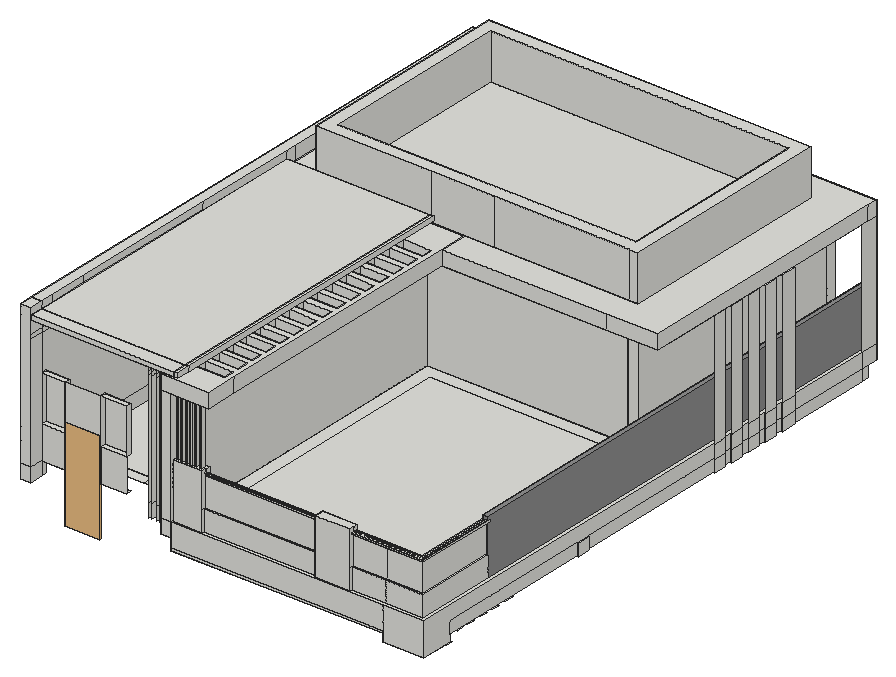
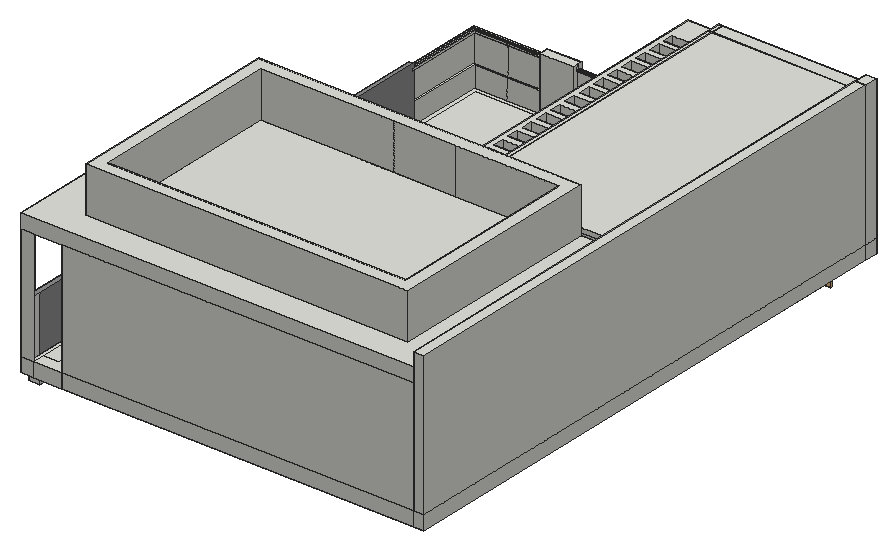
# SketchUp Ruby script. Lengths in inches.
U = 1.inch
M = Sketchup.active_model
def pt(a) = Geom::Point3d.new(a.map { |v| v * U })
def face(e, loops, mat)
  f = e.add_face(loops[0].map { |a| pt(a) })
  loops[1..].each { |l| e.add_face(l.map { |a| pt(a) }).erase! }
  f.material = f.back_material = mat if mat
  f
end
# faces: each face lists its corners as indices into pts; further lists are holes
def faces(e, pts, list, mat = nil) = list.each { |f| face(e, (f[0].is_a?(Array) ? f : [f]).map { |l| l.map { |i| pts[i] } }, mat) }
# xy, xz, yz: faces in a plane at the given z, y or x. An outline is a flat list of corners, or four numbers for a rectangle; further outlines are holes
def ring(l) = l.size == 4 ? [[l[0], l[1]], [l[2], l[1]], [l[2], l[3]], [l[0], l[3]]] : l.each_slice(2).to_a
def flat(e, list, mat, &to3) = list.each { |f| face(e, (f[0].is_a?(Array) ? f : [f]).map { |l| ring(l).map { |u, v| to3.(u, v) } }, mat) }
def xy(e, z, list, mat = nil) = flat(e, list, mat) { |x, y| [x, y, z] }
def xz(e, y, list, mat = nil) = flat(e, list, mat) { |x, z| [x, y, z] }
def yz(e, x, list, mat = nil) = flat(e, list, mat) { |y, z| [x, y, z] }
def lines(e, pts, list) = list.each { |a, b| e.add_line(pt(pts[a]), pt(pts[b])) }
# prism: a flat outline (further loops are holes) pulled along v
def prism(e, loops, v, mat = nil)
  f = face(e, loops, mat); d = Geom::Vector3d.new(v.map { |x| x * U })
  f.pushpull(f.normal.samedirection?(d) ? d.length : -d.length)
end
def box(e, o, s, mat = nil) = prism(e, [[o, [o[0] + s[0], o[1], o[2]], [o[0] + s[0], o[1] + s[1], o[2]], [o[0], o[1] + s[1], o[2]]]], [0, 0, s[2]], mat)
def at(x, y, z, deg = 0) = Geom::Transformation.translation(pt([x, y, z])) * Geom::Transformation.rotation(ORIGIN, Z_AXIS, deg.degrees)
def axes(o, x, y, z) = Geom::Transformation.new([*x, 0, *y, 0, *z, 0, *pt(o).to_a, 1])
def part(name) = M.definitions.add(name)
# library, detail: a bought-in or finely detailed component or shape, given as its bounding box
def library(name, o, s) = part(name).tap { |d| box(d.entities, o, s) }
def detail(e, o, s) = box(e.add_group.entities, o, s)
def put(e, d, t, mat = nil) = e.add_instance(d, t).tap { |i| i.material = mat if mat }
def group(e, t, mat = nil) = e.add_group.tap { |g| g.transformation = t; g.material = mat if mat }.entities
root = M.entities
M.materials.add("[Color M04]").color = [142, 142, 142]
c1 = library("c103.dxf",[0,0,0],[4.7,1.18,0.06])
xy(root,216,[[117,47.75,165,56.75],[201,47.75,261,56.75],[306,160,315,220],[306,256,315,304],[306,393.91,315,441.91]])
xy(root,235.625,[[315,0,315,9.8125,341.1875,9.8125,341.1875,28.05,341.78,28.05,341.78,23.68,351,23.68,351,0],[341.78,23.68,351,28.05],[351,23.68,352.3125,23.68,352.3125,28.93,341.78,28.93,341.78,28.05,351,28.05]])
xy(root,241.9375,[[341.1875,28.05,341.1875,482.75,351,482.75,351,401.04,352.3125,401.04,352.3125,388.24,351,388.24,351,380.51,352.3125,380.51,352.3125,369.53,351,369.53,351,362.89,352.3125,362.89,352.3125,351.72,351,351.72,351,343.76,352.3125,343.76,352.3125,332.62,351,332.62,351,325.96,352.3125,325.96,352.3125,314.875,351,314.875,351,177.375,352.3125,177.375,352.3125,166.56,351,166.56,351,94.89,341.78,94.89,341.78,87.35,351,87.35,351,79.37,341.78,79.37,341.78,73.23,351,73.23,351,66.7,341.78,66.7,341.78,60.24,351,60.24,351,52.82,341.78,52.82,341.78,46.18,351,46.18,351,41.08,341.78,41.08,341.78,35.09,351,35.09,351,28.05],[341.78,35.09,351,41.08],[351,35.09,352.3125,41.08],[341.78,46.18,351,52.82],[351,46.18,352.3125,52.82],
  [341.78,60.24,351,66.7],[351,60.24,352.3125,66.7],[341.78,73.23,351,79.37],[351,73.23,352.3125,79.37],[341.78,87.35,351,94.89],
  [351,87.35,352.3125,94.89]])
xy(root,242,[[131.25,0,315,9.8125]])
xy(root,244,[[131.25,0,315,9.8125]])
xy(root,252,[[0,0,9,11.75],[122.25,0,131.25,11.75],[131.25,9.8125,131.25,11.75,132.375,11.75,132.375,22.5,131.25,22.5,131.25,47.75,315,47.75,315,482.75,341.1875,482.75,341.1875,472.9375,324.8125,472.9375,324.8125,37.9375,141.0625,37.9375,141.0625,32.3125,142.1875,32.3125,142.1875,9.8125],[142.1875,9.8125,142.1875,32.3125,141.0625,32.3125,141.0625,37.9375,324.8125,37.9375,324.8125,472.9375,341.1875,472.9375,341.1875,9.8125],[122.25,11.75,125.16,16.5625],
  [131.25,11.75,132.375,22.5],[341.1875,28.05,351,28.05,351,314.875,352.3125,314.875,352.3125,325.96,351,325.96,351,332.62,352.3125,332.62,352.3125,343.76,351,343.76,351,351.72,352.3125,351.72,352.3125,362.89,351,362.89,351,369.53,352.3125,369.53,352.3125,380.51,351,380.51,351,388.24,352.3125,388.24,352.3125,401.04,351,401.04,351,482.75,341.1875,482.75],[0,47.75,69,56.75],[69,47.75,131.25,56.75],[131.25,47.75,315,56.75],
  [0,56.75,69,56.81],[69,56.75,78,482.75],[78,56.75,78,482.75,306,482.75,306,278.1875,131.25,278.1875,131.25,56.75],[131.25,56.75,306,278.1875],[306,56.75,315,278.1875],
  [0,56.81,69,187.47],[351,166.56,352.3125,177.375],[0,187.47,69,482.75],[306,278.1875,315,482.75],[0,482.75,69,491.75],
  [69,482.75,315,491.75],[315,482.75,351,491.75]])
xy(root,252.9375,[[341.78,166.56,345.03,166.56,341.78,177.375]])
xy(root,264,[[0,0,9,11.75],[122.25,0,131.25,11.75],[131.25,0,351,0,351,314.875,352.3125,314.875,352.3125,325.96,351,325.96,351,332.62,352.3125,332.62,352.3125,343.76,351,343.76,351,351.72,352.3125,351.72,352.3125,362.89,351,362.89,351,369.53,352.3125,369.53,352.3125,380.51,351,380.51,351,388.24,352.3125,388.24,352.3125,401.04,351,401.04,351,491.75,339.5,491.75,339.5,11.5,143.875,11.5,132.375,11.75,131.25,11.75,131.25,8.15,143.83,7.95,143.83,9.89,156.7,9.89,156.7,7.95,255.15,7.95,255.15,9.89,285.07,9.89,285.07,7.95,343.05,7.95,343.05,488.2,347.45,488.2,347.45,3.55,285.07,3.55,285.07,1.61,255.15,1.61,255.15,3.55,156.7,3.55,156.7,1.61,131.25,1.61],[131.25,1.61,131.25,8.15,143.83,7.95,143.83,9.89,156.7,9.89,156.7,7.95,255.15,7.95,255.15,9.89,285.07,9.89,285.07,7.95,343.05,7.95,343.05,73.86,347.45,73.86,347.45,3.55,285.07,3.55,285.07,1.61,255.15,1.61,255.15,3.55,156.7,3.55,156.7,1.61],[143.875,11.5,143.875,34,142.75,34,142.75,266.6875,326.5,266.6875,326.5,480.25,339.5,480.25,339.5,491.75,315,491.75,315,278.1875,131.25,278.1875,131.25,22.5,132.375,22.5,132.375,11.75],
  [143.875,11.5,339.5,11.5,339.5,480.25,326.5,480.25,326.5,266.6875,142.75,266.6875,142.75,34,143.875,34],[9,11.75,29.4,16.5625],[60.19,11.75,82.8125,16.5625],[122.25,11.75,131.25,22.5],[131.25,11.75,132.375,22.5],
  [122.25,22.5,131.25,278.1875],[343.05,73.86,347.45,488.2],[9,278.1875,306,287.1875],[306,278.1875,315,482.75],[9,482.75,315,491.75]])
xy(root,282,[[156.7,3.55,255.15,5.09],[285.07,3.55,347.45,3.55,347.45,73.86,345.91,73.86,345.91,5.09,285.07,5.09],[156.7,6.41,255.15,7.95],[285.07,6.41,344.59,6.41,344.59,73.86,343.05,73.86,343.05,7.95,285.07,7.95]])
xy(root,292.85,[[9,11.75,29.4,16.5625],[60.19,11.75,82.8125,16.5625]])
xy(root,307.3125,[[[283.34,3.36,283.34,8.14,342.86,8.14,342.86,75.59,347.64,75.59,347.64,3.36],[285.07,5.09,345.91,5.09,345.91,73.86,344.59,73.86,344.59,6.41,285.07,6.41]],[[155.89,4.28,255.96,7.22],[156.7,5.09,255.15,6.41]],[156.7,5.09,255.15,6.41],[285.07,5.09,285.07,6.41,344.59,6.41,344.59,73.86,345.91,73.86,345.91,5.09]])
xy(root,308.625,[[[283.34,3.36,347.64,3.36,347.64,75.59,342.86,75.59,342.86,8.14,283.34,8.14],[285.07,5.09,285.07,6.41,344.59,6.41,344.59,73.86,345.91,73.86,345.91,5.09]],[[155.89,4.28,255.96,7.22],[156.7,5.09,255.15,6.41]],[156.7,5.09,255.15,6.41],[285.07,5.09,345.91,5.09,345.91,73.86,344.59,73.86,344.59,6.41,285.07,6.41]])
xy(root,312,[[[131.25,1.61,156.7,1.61,156.7,9.89,143.83,9.89,143.83,7.95,131.25,8.15],[132.875,3.73,135.0625,7.27],[136.5,3.73,138.6875,7.27],[140.5625,3.73,142.75,7.27],[144.5,3.73,146.6875,7.27],[148.5,3.73,150.6875,7.27],[152.875,3.73,155.0625,7.27]],[255.15,1.61,285.07,9.89],[132.875,3.73,135.0625,7.27],[136.5,3.73,138.6875,7.27],[140.5625,3.73,142.75,7.27],
  [144.5,3.73,146.6875,7.27],[148.5,3.73,150.6875,7.27],[152.875,3.73,155.0625,7.27]])
xy(root,312,[[343.05,73.86,347.45,488.2]],"[Color M04]")
xy(root,332.24,[[9,11.75,29.4,16.5625],[60.19,11.75,82.8125,16.5625]])
xy(root,363.8125,[[122.25,0,131.25,278.1875],[[131.25,0,131.25,27.62,133.86,27.62,133.86,23.53,158.62,23.53,158.62,27.62,163.5625,27.62,163.5625,0],[152.875,3.73,155.0625,7.27],[144.5,3.73,146.6875,7.27],[148.5,3.73,150.6875,7.27],[140.5625,3.73,142.75,7.27],[136.5,3.73,138.6875,7.27],[132.875,3.73,135.0625,7.27]],[[131.25,27.62,131.25,278.1875,163.5625,278.1875,163.5625,27.62,158.62,27.62,158.62,33.15,133.86,33.15,133.86,27.62],[133.86,38.59,158.62,48.21],[133.86,53.65,158.62,63.28],[133.86,68.71,158.62,78.34],[133.86,83.78,158.62,93.4],[133.86,99.28,158.62,108.9],[133.86,114.78,158.62,124.4],[133.86,223.28,158.62,232.9],[133.86,207.78,158.62,217.4],[133.86,176.78,158.62,186.4],[133.86,130.28,158.62,139.9],[133.86,161.28,158.62,170.9],[133.86,238.78,158.62,248.4],[133.86,192.28,158.62,201.9],[133.86,145.78,158.62,155.4]],[163.5625,254.0625,306,278.1875],[306,254.0625,351,278.1875],
  [9,278.1875,306,287.1875],[306,278.1875,315,482.75],[315,278.1875,315,482.75,339.69,482.75,339.69,482.53,341.78,482.53,341.78,475.81,351,475.81,351,401.04,341.78,401.04,341.78,388.24,351,388.24,351,380.51,341.78,380.51,341.78,369.53,351,369.53,351,362.89,341.78,362.89,341.78,351.72,351,351.72,351,343.76,341.78,343.76,341.78,332.62,351,332.62,351,325.96,341.78,325.96,341.78,314.875,351,314.875,351,278.1875],[9,287.1875,306,482.75],[351,314.875,352.3125,325.96],
  [351,332.62,352.3125,343.76],[351,351.72,352.3125,362.89],[351,369.53,352.3125,380.51],[351,388.24,352.3125,401.04],[341.78,475.81,351,475.81,351,482.75,339.69,482.75,339.69,482.53,341.78,482.53],
  [9,482.75,315,491.75],[315,482.75,339.69,491.75],[339.69,482.75,351,491.75]])
xy(root,376.25,[[122.25,0,133.86,11.75],[133.86,0,163.5625,0,163.5625,278.1875,133.86,278.1875,133.86,248.4,158.62,248.4,158.62,238.78,133.86,238.78,133.86,232.9,158.62,232.9,158.62,223.28,133.86,223.28,133.86,217.4,158.62,217.4,158.62,207.78,133.86,207.78,133.86,201.9,158.62,201.9,158.62,192.28,133.86,192.28,133.86,186.4,158.62,186.4,158.62,176.78,133.86,176.78,133.86,170.9,158.62,170.9,158.62,161.28,133.86,161.28,133.86,155.4,158.62,155.4,158.62,145.78,133.86,145.78,133.86,139.9,158.62,139.9,158.62,130.28,133.86,130.28,133.86,124.4,158.62,124.4,158.62,114.78,133.86,114.78,133.86,108.9,158.62,108.9,158.62,99.28,133.86,99.28,133.86,93.4,158.62,93.4,158.62,83.78,133.86,83.78,133.86,78.34,158.62,78.34,158.62,68.71,133.86,68.71,133.86,63.28,158.62,63.28,158.62,53.65,133.86,53.65,133.86,48.21,158.62,48.21,158.62,38.59,133.86,38.59,133.86,33.15,158.62,33.15,158.62,23.53,133.86,23.53],[[163.5625,254.0625,351,254.0625,351,491.75,9,491.75,9,278.1875,163.5625,278.1875],[33.8125,278.875,314.3125,466.9375]],[[33.8125,278.875,314.3125,466.9375],[44.48,289.54,303.64,456.27]],[44.48,289.54,303.64,456.27]])
xy(root,378.375,[[9,0,122.25,11.75],[122.25,0,133.86,11.75],[133.86,0,137.04,11.75],[9,11.75,9,22.5,122.25,22.5,122.25,11.75,117.62,11.75,117.62,16.5625,115.5625,16.5625,115.5625,11.75,111.75,11.75,111.75,16.5625,109.5,16.5625,109.5,11.75,105.0625,11.75,105.0625,16.5625,102.625,16.5625,102.625,11.75],[102.625,11.75,105.0625,16.5625],
  [109.5,11.75,111.75,16.5625],[115.5625,11.75,117.62,16.5625],[122.25,11.75,133.86,278.1875],[133.86,11.75,137.04,278.1875],[9,22.5,122.25,278.1875]])
xy(root,382.375,[[9,0,133.86,11.75],[133.86,0,137.04,11.75],[9,11.75,133.86,278.1875],[133.86,11.75,137.04,278.1875]])
xy(root,388.3125,[[0,0,9,11.75],[0,11.75,9,491.75]])
xy(root,416.0625,[[[33.8125,278.875,314.3125,466.9375],[44.48,289.54,303.64,456.27]]])
xz(root,0,[[315,235.625,351,264],[131.25,242,315,244],[131.25,244,315,264],[0,252,9,264],[122.25,252,131.25,264],
  [0,264,9,388.3125],[122.25,264,131.25,363.8125],[122.25,363.8125,163.5625,376.25],[9,378.375,133.86,382.375],[133.86,378.375,137.04,382.375]])
xz(root,1.61,[[131.25,264,156.7,312],[255.15,264,285.07,312]])
xz(root,3.36,[[283.34,307.3125,315,308.625],[315,307.3125,347.64,308.625]])
xz(root,3.55,[[156.7,264,255.15,282],[285.07,264,315,282],[315,264,347.45,282]])
xz(root,3.73,[[132.875,312,135.0625,363.8125],[136.5,312,138.6875,363.8125],[140.5625,312,142.75,363.8125],[144.5,312,146.6875,363.8125],[148.5,312,150.6875,363.8125],
  [152.875,312,155.0625,363.8125]])
xz(root,4.28,[[155.89,307.3125,255.96,308.625]])
xz(root,5.09,[[156.7,282,255.15,307.3125],[285.07,282,315,307.3125],[315,282,345.91,307.3125],[156.7,307.3125,255.15,308.625],[285.07,307.3125,315,308.625],
  [315,307.3125,345.91,308.625]])
xz(root,6.41,[[156.7,282,255.15,307.3125],[285.07,282,315,307.3125],[315,282,344.59,307.3125],[156.7,307.3125,255.15,308.625],[285.07,307.3125,315,308.625],
  [315,307.3125,344.59,308.625]])
xz(root,7.22,[[155.89,307.3125,255.96,308.625]])
xz(root,7.27,[[132.875,312,135.0625,363.8125],[136.5,312,138.6875,363.8125],[140.5625,312,142.75,363.8125],[144.5,312,146.6875,363.8125],[148.5,312,150.6875,363.8125],
  [152.875,312,155.0625,363.8125]])
xz(root,7.95,[[156.7,264,255.15,282],[285.07,264,315,282],[315,264,343.05,282]])
xz(root,8.14,[[283.34,307.3125,315,308.625],[315,307.3125,342.86,308.625]])
xz(root,9.8125,[[315,235.625,341.1875,252],[131.25,242,142.1875,244],[142.1875,242,315,244],[131.25,244,142.1875,252],[142.1875,244,315,252]])
xz(root,9.89,[[143.83,264,156.7,312],[255.15,264,285.07,312]])
xz(root,11.75,[[0,252,9,264],[122.25,252,131.25,264],[131.25,252,132.375,264],[0,264,9,388.3125],[9,264,29.4,292.85],
  [29.4,264,60.19,292.85],[60.19,264,82.8125,292.85],[29.4,292.85,60.19,332.24],[122.25,376.25,133.86,378.375],[9,378.375,133.86,382.375],
  [133.86,378.375,137.04,382.375]])
xz(root,16.5625,[[9,292.85,29.4,332.24],[60.19,292.85,82.8125,332.24]])
xz(root,22.5,[[131.25,252,132.375,264],[9,363.8125,122.25,367],[9,367,122.25,378.375]])
xz(root,23.53,[[133.86,363.8125,158.62,376.25]])
xz(root,28.05,[[341.1875,235.625,351,241.9375],[341.1875,241.9375,351,252]])
xz(root,33.15,[[133.86,363.8125,158.62,376.25]])
xz(root,38.59,[[133.86,363.8125,158.62,376.25]])
xz(root,48.21,[[133.86,363.8125,158.62,376.25]])
xz(root,53.65,[[133.86,363.8125,158.62,376.25]])
xz(root,63.28,[[133.86,363.8125,158.62,376.25]])
xz(root,68.71,[[133.86,363.8125,158.62,376.25]])
xz(root,73.86,[[343.05,264,347.45,264,347.45,282,345.91,282,345.91,307.3125,344.59,307.3125,344.59,282,343.05,282],[344.59,307.3125,345.91,308.625]])
xz(root,73.86,[[343.05,282,344.59,282,344.59,308.625,345.91,308.625,345.91,282,347.45,282,347.45,312,343.05,312]],"[Color M04]")
xz(root,75.59,[[342.86,307.3125,347.64,308.625]])
xz(root,78.34,[[133.86,363.8125,158.62,376.25]])
xz(root,83.78,[[133.86,363.8125,158.62,376.25]])
xz(root,93.4,[[133.86,363.8125,158.62,376.25]])
xz(root,99.28,[[133.86,363.8125,158.62,376.25]])
xz(root,108.9,[[133.86,363.8125,158.62,376.25]])
xz(root,114.78,[[133.86,363.8125,158.62,376.25]])
xz(root,124.4,[[133.86,363.8125,158.62,376.25]])
xz(root,130.28,[[133.86,363.8125,158.62,376.25]])
xz(root,139.9,[[133.86,363.8125,158.62,376.25]])
xz(root,145.78,[[133.86,363.8125,158.62,376.25]])
xz(root,155.4,[[133.86,363.8125,158.62,376.25]])
xz(root,161.28,[[133.86,363.8125,158.62,376.25]])
xz(root,166.56,[[351,241.9375,352.3125,252]])
xz(root,170.9,[[133.86,363.8125,158.62,376.25]])
xz(root,176.78,[[133.86,363.8125,158.62,376.25]])
xz(root,177.375,[[351,241.9375,352.3125,252]])
xz(root,186.4,[[133.86,363.8125,158.62,376.25]])
xz(root,192.28,[[133.86,363.8125,158.62,376.25]])
xz(root,201.9,[[133.86,363.8125,158.62,376.25]])
xz(root,207.78,[[133.86,363.8125,158.62,376.25]])
xz(root,217.4,[[133.86,363.8125,158.62,376.25]])
xz(root,223.28,[[133.86,363.8125,158.62,376.25]])
xz(root,232.9,[[133.86,363.8125,158.62,376.25]])
xz(root,238.78,[[133.86,363.8125,158.62,376.25]])
xz(root,248.4,[[133.86,363.8125,158.62,376.25]])
xz(root,254.0625,[[163.5625,363.8125,306,376.25],[306,363.8125,351,376.25]])
xz(root,278.1875,[[131.25,252,306,264],[306,252,315,264],[9,264,122.25,363.8125],[122.25,264,131.25,363.8125],[131.25,264,306,363.8125],
  [306,264,315,363.8125],[9,363.8125,122.25,376.25],[122.25,363.8125,163.5625,376.25],[122.25,376.25,133.86,378.375],[9,378.375,133.86,382.375],
  [133.86,378.375,137.04,382.375]])
xz(root,278.875,[[33.8125,376.25,133.86,416.0625],[133.86,376.25,188.375,416.0625],[188.375,376.25,306,416.0625],[306,376.25,314.3125,416.0625]])
xz(root,287.1875,[[9,264,306,363.8125]])
xz(root,289.54,[[44.48,376.25,133.86,416.0625],[133.86,376.25,188.375,416.0625],[188.375,376.25,303.64,416.0625]])
xz(root,314.875,[[351,241.9375,352.3125,252],[351,252,352.3125,264]])
xz(root,325.96,[[351,241.9375,352.3125,252],[351,252,352.3125,264]])
xz(root,332.62,[[351,241.9375,352.3125,252],[351,252,352.3125,264]])
xz(root,343.76,[[351,241.9375,352.3125,252],[351,252,352.3125,264]])
xz(root,351.72,[[351,241.9375,352.3125,252],[351,252,352.3125,264]])
xz(root,362.89,[[351,241.9375,352.3125,252],[351,252,352.3125,264]])
xz(root,369.53,[[351,241.9375,352.3125,252],[351,252,352.3125,264]])
xz(root,380.51,[[351,241.9375,352.3125,252],[351,252,352.3125,264]])
xz(root,388.24,[[351,241.9375,352.3125,252],[351,252,352.3125,264]])
xz(root,401.04,[[351,241.9375,352.3125,252],[351,252,352.3125,264]])
xz(root,456.27,[[44.48,376.25,303.64,416.0625]])
xz(root,466.9375,[[33.8125,376.25,314.3125,416.0625]])
xz(root,482.75,[[341.1875,241.9375,351,252],[9,264,306,363.8125],[306,264,315,363.8125]])
xz(root,488.2,[[343.05,264,347.45,312]])
xz(root,491.75,[[0,252,9,264],[9,252,315,264],[315,252,339.69,264],[339.69,252,351,264],[0,264,9,388.3125],
  [9,264,315,363.8125],[339.69,264,351,363.8125],[9,363.8125,351,376.25]])
yz(root,0,[[0,252,11.75,264],[11.75,252,491.75,264],[0,264,11.75,388.3125],[11.75,264,491.75,388.3125]])
yz(root,9,[[0,252,11.75,264],[11.75,252,16.5625,264],[0,264,11.75,363.8125],[278.1875,264,287.1875,363.8125],[482.75,264,491.75,363.8125],
  [11.75,292.85,16.5625,332.24],[0,363.8125,11.75,367],[11.75,363.8125,22.5,367],[278.1875,363.8125,287.1875,376.25],[287.1875,363.8125,491.75,376.25],
  [0,367,11.75,378.375],[11.75,367,22.5,378.375],[278.1875,376.25,287.1875,388.3125],[287.1875,376.25,482.75,388.3125],[482.75,376.25,491.75,388.3125],
  [0,378.375,11.75,382.375],[11.75,378.375,22.5,382.375],[22.5,378.375,56.81,382.375],[56.81,378.375,187.47,382.375],[187.47,378.375,278.1875,382.375],
  [0,382.375,11.75,388.3125],[11.75,382.375,22.5,388.3125],[22.5,382.375,56.81,388.3125],[56.81,382.375,187.47,388.3125],[187.47,382.375,278.1875,388.3125]])
yz(root,29.4,[[11.75,292.85,16.5625,332.24]])
yz(root,33.8125,[[278.875,376.25,466.9375,416.0625]])
yz(root,44.48,[[289.54,376.25,456.27,416.0625]])
yz(root,60.19,[[11.75,292.85,16.5625,332.24]])
yz(root,82.8125,[[11.75,292.85,16.5625,332.24]])
yz(root,102.625,[[11.75,252,16.5625,264],[11.75,264,16.5625,363.8125],[11.75,363.8125,16.5625,367],[11.75,367,16.5625,376.25],[11.75,376.25,16.5625,378.375]])
yz(root,105.0625,[[11.75,252,16.5625,264],[11.75,264,16.5625,363.8125],[11.75,363.8125,16.5625,367],[11.75,367,16.5625,376.25],[11.75,376.25,16.5625,378.375]])
yz(root,109.5,[[11.75,252,16.5625,264],[11.75,264,16.5625,363.8125],[11.75,363.8125,16.5625,367],[11.75,367,16.5625,376.25],[11.75,376.25,16.5625,378.375]])
yz(root,111.75,[[11.75,252,16.5625,264],[11.75,264,16.5625,363.8125],[11.75,363.8125,16.5625,367],[11.75,367,16.5625,376.25],[11.75,376.25,16.5625,378.375]])
yz(root,115.5625,[[11.75,252,16.5625,264],[11.75,264,16.5625,363.8125],[11.75,363.8125,16.5625,367],[11.75,367,16.5625,376.25],[11.75,376.25,16.5625,378.375]])
yz(root,122.25,[[0,252,11.75,264],[0,264,11.75,363.8125],[11.75,264,22.5,363.8125],[22.5,264,278.1875,363.8125],[0,363.8125,11.75,367],
  [11.75,363.8125,22.5,367],[22.5,363.8125,278.1875,378.375],[0,367,11.75,376.25],[11.75,367,22.5,378.375]])
yz(root,131.25,[[0,242,9.8125,244],[0,244,9.8125,252],[0,252,11.75,264],[11.75,252,22.5,264],[22.5,252,27.62,264],
  [27.62,252,278.1875,264],[0,264,1.61,264,1.61,312,8.15,312,8.15,264,27.62,264,27.62,363.8125,0,363.8125],[1.61,264,8.15,312],[27.62,264,278.1875,363.8125]])
yz(root,132.375,[[11.75,252,22.5,264]])
yz(root,132.875,[[3.73,312,7.27,363.8125]])
yz(root,133.86,[[23.53,363.8125,33.15,376.25],[38.59,363.8125,48.21,376.25],[53.65,363.8125,63.28,376.25],[68.71,363.8125,78.34,376.25],[83.78,363.8125,93.4,376.25],
  [99.28,363.8125,108.9,376.25],[114.78,363.8125,124.4,376.25],[130.28,363.8125,139.9,376.25],[145.78,363.8125,155.4,376.25],[161.28,363.8125,170.9,376.25],
  [176.78,363.8125,186.4,376.25],[192.28,363.8125,201.9,376.25],[207.78,363.8125,217.4,376.25],[223.28,363.8125,232.9,376.25],[238.78,363.8125,248.4,376.25],
  [11.75,376.25,278.1875,378.375],[0,378.375,11.75,382.375],[11.75,378.375,278.1875,382.375]])
yz(root,135.0625,[[3.73,312,7.27,363.8125]])
yz(root,136.5,[[3.73,312,7.27,363.8125]])
yz(root,137.04,[[0,378.375,11.75,382.375],[11.75,378.375,278.1875,382.375]])
yz(root,138.6875,[[3.73,312,7.27,363.8125]])
yz(root,140.5625,[[3.73,312,7.27,363.8125]])
yz(root,142.75,[[3.73,312,7.27,363.8125]])
yz(root,143.83,[[7.95,264,9.89,312]])
yz(root,144.5,[[3.73,312,7.27,363.8125]])
yz(root,146.6875,[[3.73,312,7.27,363.8125]])
yz(root,148.5,[[3.73,312,7.27,363.8125]])
yz(root,150.6875,[[3.73,312,7.27,363.8125]])
yz(root,152.875,[[3.73,312,7.27,363.8125]])
yz(root,155.0625,[[3.73,312,7.27,363.8125]])
yz(root,155.89,[[4.28,307.3125,7.22,308.625]])
yz(root,156.7,[[1.61,264,3.55,282],[7.95,264,9.89,282],[1.61,282,5.09,312],[6.41,282,9.89,312],[5.09,307.3125,6.41,308.625],
  [5.09,308.625,6.41,312]])
yz(root,158.62,[[23.53,363.8125,33.15,376.25],[38.59,363.8125,48.21,376.25],[53.65,363.8125,63.28,376.25],[68.71,363.8125,78.34,376.25],[83.78,363.8125,93.4,376.25],
  [99.28,363.8125,108.9,376.25],[114.78,363.8125,124.4,376.25],[130.28,363.8125,139.9,376.25],[145.78,363.8125,155.4,376.25],[161.28,363.8125,170.9,376.25],
  [176.78,363.8125,186.4,376.25],[192.28,363.8125,201.9,376.25],[207.78,363.8125,217.4,376.25],[223.28,363.8125,232.9,376.25],[238.78,363.8125,248.4,376.25]])
yz(root,163.5625,[[0,363.8125,27.62,376.25],[27.62,363.8125,254.0625,376.25],[254.0625,363.8125,278.1875,376.25]])
yz(root,255.15,[[1.61,264,3.55,282],[7.95,264,9.89,282],[1.61,282,5.09,312],[6.41,282,9.89,312],[5.09,307.3125,6.41,308.625],
  [5.09,308.625,6.41,312]])
yz(root,255.96,[[4.28,307.3125,7.22,308.625]])
yz(root,283.34,[[3.36,307.3125,8.14,308.625]])
yz(root,285.07,[[1.61,264,3.55,282],[7.95,264,9.89,282],[1.61,282,5.09,312],[6.41,282,9.89,312],[5.09,307.3125,6.41,308.625],
  [5.09,308.625,6.41,312]])
yz(root,303.64,[[289.54,376.25,456.27,416.0625]])
yz(root,306,[[278.1875,264,287.1875,363.8125],[287.1875,264,482.75,363.8125]])
yz(root,314.3125,[[278.875,376.25,466.9375,416.0625]])
yz(root,315,[[0,235.625,9.8125,242],[0,242,9.8125,244],[278.1875,252,482.75,264],[482.75,252,491.75,264],[278.1875,264,482.75,363.8125],
  [482.75,264,491.75,363.8125]])
yz(root,341.1875,[[9.8125,235.625,28.05,252],[28.05,241.9375,472.9375,252],[472.9375,241.9375,482.75,252]])
yz(root,342.86,[[8.14,307.3125,75.59,308.625]])
yz(root,343.05,[[7.95,264,73.86,282],[480.25,264,488.2,312]])
yz(root,343.05,[[73.86,264,480.25,312]],"[Color M04]")
yz(root,344.59,[[6.41,282,73.86,307.3125],[6.41,307.3125,73.86,308.625]])
yz(root,345.91,[[5.09,282,73.86,307.3125],[5.09,307.3125,73.86,308.625]])
yz(root,347.45,[[3.55,264,73.86,282]])
yz(root,347.45,[[73.86,264,488.2,312]],"[Color M04]")
yz(root,347.64,[[3.36,307.3125,75.59,308.625]])
yz(root,351,[[0,235.625,28.05,235.625,28.05,252,314.875,252,314.875,264,0,264],[28.05,241.9375,166.56,252],[177.375,241.9375,314.875,252],[325.96,241.9375,332.62,252],[343.76,241.9375,351.72,252],
  [362.89,241.9375,369.53,252],[380.51,241.9375,388.24,252],[401.04,241.9375,475.81,252],[475.81,241.9375,482.75,252],[325.96,252,332.62,264],
  [343.76,252,351.72,264],[362.89,252,369.53,264],[380.51,252,388.24,264],[401.04,252,475.81,264],[475.81,252,491.75,264],
  [475.81,264,491.75,363.8125],[254.0625,363.8125,482.75,376.25],[482.75,363.8125,491.75,376.25]])
yz(root,352.3125,[[166.56,241.9375,177.375,252],[314.875,241.9375,325.96,252],[332.62,241.9375,343.76,252],[351.72,241.9375,362.89,252],[369.53,241.9375,380.51,252],
  [388.24,241.9375,401.04,252],[314.875,252,325.96,264],[332.62,252,343.76,264],[351.72,252,362.89,264],[369.53,252,380.51,264],
  [388.24,252,401.04,264],[314.875,264,325.96,363.8125],[332.62,264,343.76,363.8125],[351.72,264,362.89,363.8125],[369.53,264,380.51,363.8125],
  [388.24,264,401.04,363.8125]])
p = [[351,177.375,252],[341.78,177.375,252.9375],[345.03,166.56,252.9375],[348.3,166.56,252.9375],[351,166.56,252],[143.83,7.95,264],
  [131.25,8.15,264],[131.25,8.15,312],[143.83,7.95,312],[306,482.75,363.8125],[306,482.75,376.25],[306,287.1875,363.8125],
  [306,287.1875,376.25]]
faces(root,p,[[0,1,2],[3,0,2],[4,0,3],[5,6,7,8]])
lines(root,p,[[9,10],[11,12]])
put(root,c1,axes([29.43,11.22,220.51],[0,0,17.238],[26.0445,0,0],[0,17.238,0]))
